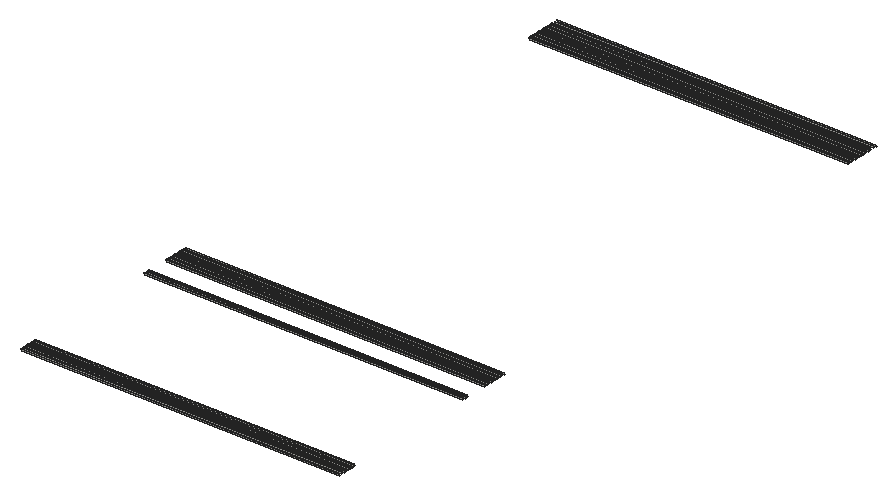
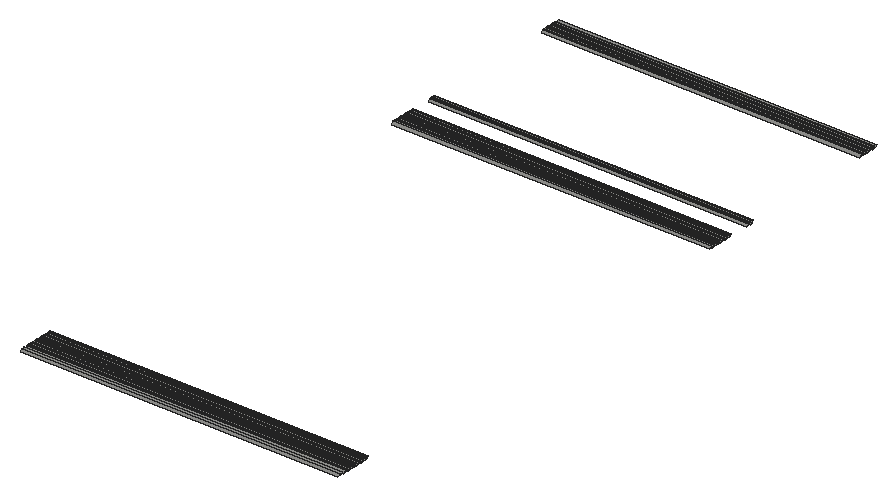
# SketchUp Ruby script. Lengths in inches.
U = 1.inch
M = Sketchup.active_model
def pt(a) = Geom::Point3d.new(a.map { |v| v * U })
def face(e, loops, mat)
  f = e.add_face(loops[0].map { |a| pt(a) })
  loops[1..].each { |l| e.add_face(l.map { |a| pt(a) }).erase! }
  f.material = f.back_material = mat if mat
  f
end
# faces: each face lists its corners as indices into pts; further lists are holes
def faces(e, pts, list, mat = nil) = list.each { |f| face(e, (f[0].is_a?(Array) ? f : [f]).map { |l| l.map { |i| pts[i] } }, mat) }
# xy, xz, yz: faces in a plane at the given z, y or x. An outline is a flat list of corners, or four numbers for a rectangle; further outlines are holes
def ring(l) = l.size == 4 ? [[l[0], l[1]], [l[2], l[1]], [l[2], l[3]], [l[0], l[3]]] : l.each_slice(2).to_a
def flat(e, list, mat, &to3) = list.each { |f| face(e, (f[0].is_a?(Array) ? f : [f]).map { |l| ring(l).map { |u, v| to3.(u, v) } }, mat) }
def xy(e, z, list, mat = nil) = flat(e, list, mat) { |x, y| [x, y, z] }
def xz(e, y, list, mat = nil) = flat(e, list, mat) { |x, z| [x, y, z] }
def yz(e, x, list, mat = nil) = flat(e, list, mat) { |y, z| [x, y, z] }
def lines(e, pts, list) = list.each { |a, b| e.add_line(pt(pts[a]), pt(pts[b])) }
# prism: a flat outline (further loops are holes) pulled along v
def prism(e, loops, v, mat = nil)
  f = face(e, loops, mat); d = Geom::Vector3d.new(v.map { |x| x * U })
  f.pushpull(f.normal.samedirection?(d) ? d.length : -d.length)
end
def box(e, o, s, mat = nil) = prism(e, [[o, [o[0] + s[0], o[1], o[2]], [o[0] + s[0], o[1] + s[1], o[2]], [o[0], o[1] + s[1], o[2]]]], [0, 0, s[2]], mat)
def at(x, y, z, deg = 0) = Geom::Transformation.translation(pt([x, y, z])) * Geom::Transformation.rotation(ORIGIN, Z_AXIS, deg.degrees)
def axes(o, x, y, z) = Geom::Transformation.new([*x, 0, *y, 0, *z, 0, *pt(o).to_a, 1])
def part(name) = M.definitions.add(name)
# library, detail: a bought-in or finely detailed component or shape, given as its bounding box
def library(name, o, s) = part(name).tap { |d| box(d.entities, o, s) }
def detail(e, o, s) = box(e.add_group.entities, o, s)
def put(e, d, t, mat = nil) = e.add_instance(d, t).tap { |i| i.material = mat if mat }
def group(e, t, mat = nil) = e.add_group.tap { |g| g.transformation = t; g.material = mat if mat }.entities
root = M.entities
c1 = part("Group452\#1")
p = [[-385.16,721.125,5.875],[385.16,721.125,5.875],[385.16,724.52,0],[-385.16,724.52,0]]
faces(c1.entities,p,[[0,1,2,3]])
c2 = part("Group453\#1")
p = [[-385.16,725.0625,5.875],[385.16,725.0625,5.875],[385.16,728.45,0],[-385.16,728.45,0]]
faces(c2.entities,p,[[0,1,2,3]])
c3 = part("Group454\#1")
p = [[-385.16,729,5.875],[385.16,729,5.875],[385.16,732.39,0],[-385.16,732.39,0]]
faces(c3.entities,p,[[0,1,2,3]])
c4 = part("Group455\#1")
p = [[-385.16,732.9375,5.875],[385.16,732.9375,5.875],[385.16,736.33,0],[-385.16,736.33,0]]
faces(c4.entities,p,[[0,1,2,3]])
c5 = part("Group456\#1")
p = [[-385.16,736.875,5.875],[385.16,736.875,5.875],[385.16,740.27,0],[-385.16,740.27,0]]
faces(c5.entities,p,[[0,1,2,3]])
c6 = part("Group457\#1")
p = [[-385.16,740.8125,5.875],[385.16,740.8125,5.875],[385.16,744.2,0],[-385.16,744.2,0]]
faces(c6.entities,p,[[0,1,2,3]])
c7 = part("Group458\#1")
p = [[385.16,748.14,0],[-385.16,748.14,0],[-385.16,744.75,5.875],[385.16,744.75,5.875]]
faces(c7.entities,p,[[0,1,2,3]])
c8 = part("Group459\#1")
p = [[-385.16,748.6875,5.875],[385.16,748.6875,5.875],[385.16,752.08,0],[-385.16,752.08,0]]
faces(c8.entities,p,[[0,1,2,3]])
c9 = part("Group460\#1")
p = [[385.16,756.02,0],[-385.16,756.02,0],[-385.16,752.625,5.875],[385.16,752.625,5.875]]
faces(c9.entities,p,[[0,1,2,3]])
c10 = part("Group461\#1")
p = [[385.16,759.95,0],[-385.16,759.95,0],[-385.16,756.5625,5.875],[385.16,756.5625,5.875]]
faces(c10.entities,p,[[0,1,2,3]])
c11 = part("Group462\#1")
p = [[-385.16,760.5,5.875],[385.16,760.5,5.875],[385.16,763.89,0],[-385.16,763.89,0]]
faces(c11.entities,p,[[0,1,2,3]])
c12 = part("Group463\#1")
p = [[-385.16,764.4375,5.875],[385.16,764.4375,5.875],[385.16,767.83,0],[-385.16,767.83,0]]
faces(c12.entities,p,[[0,1,2,3]])
c13 = part("Group464\#1")
p = [[-385.16,768.375,5.875],[385.16,768.375,5.875],[385.16,771.77,0],[-385.16,771.77,0]]
faces(c13.entities,p,[[0,1,2,3]])
c14 = part("Group465\#1")
p = [[-385.16,772.3125,5.875],[385.16,772.3125,5.875],[385.16,775.7,0],[-385.16,775.7,0]]
faces(c14.entities,p,[[0,1,2,3]])
c15 = part("Group466\#1")
p = [[385.16,779.64,0],[-385.16,779.64,0],[-385.16,776.25,5.875],[385.16,776.25,5.875]]
faces(c15.entities,p,[[0,1,2,3]])
c16 = part("Group467\#1")
p = [[385.16,783.58,0],[-385.16,783.58,0],[-385.16,780.1875,5.875],[385.16,780.1875,5.875]]
faces(c16.entities,p,[[0,1,2,3]])
c17 = part("Group468\#1")
p = [[-385.16,784.125,5.875],[385.16,784.125,5.875],[385.16,787.52,0],[-385.16,787.52,0]]
faces(c17.entities,p,[[0,1,2,3]])
c18 = part("Group469\#1")
p = [[-385.16,788.0625,5.875],[385.16,788.0625,5.875],[385.16,791.45,0],[-385.16,791.45,0]]
faces(c18.entities,p,[[0,1,2,3]])
c19 = part("Group470\#1")
p = [[-385.16,792,5.875],[385.16,792,5.875],[385.16,795.39,0],[-385.16,795.39,0]]
faces(c19.entities,p,[[0,1,2,3]])
c20 = part("Group472\#1")
p = [[385.16,803.27,0],[-385.16,803.27,0],[-385.16,799.875,5.875],[385.16,799.875,5.875]]
faces(c20.entities,p,[[0,1,2,3]])
c21 = part("Group474\#1")
p = [[-385.16,807.75,5.875],[385.16,807.75,5.875],[385.16,811.14,0],[-385.16,811.14,0]]
faces(c21.entities,p,[[0,1,2,3]])
c22 = part("Group156\#1")
p = [[385.16,-440.98,0],[-385.16,-440.98,0],[-385.16,-444.375,5.875],[385.16,-444.375,5.875]]
faces(c22.entities,p,[[0,1,2,3]])
c23 = part("Group157\#1")
p = [[-385.16,-440.4375,5.875],[385.16,-440.4375,5.875],[385.16,-437.05,0],[-385.16,-437.05,0]]
faces(c23.entities,p,[[0,1,2,3]])
c24 = part("Group158\#1")
p = [[-385.16,-436.5,5.875],[385.16,-436.5,5.875],[385.16,-433.11,0],[-385.16,-433.11,0]]
faces(c24.entities,p,[[0,1,2,3]])
c25 = part("Group159\#1")
p = [[-385.16,-432.5625,5.875],[385.16,-432.5625,5.875],[385.16,-429.17,0],[-385.16,-429.17,0]]
faces(c25.entities,p,[[0,1,2,3]])
c26 = part("Group160\#1")
p = [[385.16,-425.23,0],[-385.16,-425.23,0],[-385.16,-428.625,5.875],[385.16,-428.625,5.875]]
faces(c26.entities,p,[[0,1,2,3]])
c27 = part("Group173\#1")
p = [[-385.16,-377.4375,5.875],[385.16,-377.4375,5.875],[385.16,-374.05,0],[-385.16,-374.05,0]]
faces(c27.entities,p,[[0,1,2,3]])
c28 = part("Group174\#1")
p = [[-385.16,-373.5,5.875],[385.16,-373.5,5.875],[385.16,-370.11,0],[-385.16,-370.11,0]]
faces(c28.entities,p,[[0,1,2,3]])
c29 = part("Group175\#1")
p = [[385.16,-366.17,0],[-385.16,-366.17,0],[-385.16,-369.5625,5.875],[385.16,-369.5625,5.875]]
faces(c29.entities,p,[[0,1,2,3]])
c30 = part("Group176\#1")
p = [[-385.16,-365.625,5.875],[385.16,-365.625,5.875],[385.16,-362.23,0],[-385.16,-362.23,0]]
faces(c30.entities,p,[[0,1,2,3]])
c31 = part("Group177\#1")
p = [[385.16,-358.3,0],[-385.16,-358.3,0],[-385.16,-361.6875,5.875],[385.16,-361.6875,5.875]]
faces(c31.entities,p,[[0,1,2,3]])
c32 = part("Group178\#1")
p = [[-385.16,-357.75,5.875],[385.16,-357.75,5.875],[385.16,-354.36,0],[-385.16,-354.36,0]]
faces(c32.entities,p,[[0,1,2,3]])
c33 = part("Group179\#1")
p = [[385.16,-350.42,0],[-385.16,-350.42,0],[-385.16,-353.8125,5.875],[385.16,-353.8125,5.875]]
faces(c33.entities,p,[[0,1,2,3]])
c34 = part("Group180\#1")
p = [[385.16,-346.48,0],[-385.16,-346.48,0],[-385.16,-349.875,5.875],[385.16,-349.875,5.875]]
faces(c34.entities,p,[[0,1,2,3]])
c35 = part("Group181\#1")
p = [[-385.16,-345.9375,5.875],[385.16,-345.9375,5.875],[385.16,-342.55,0],[-385.16,-342.55,0]]
faces(c35.entities,p,[[0,1,2,3]])
c36 = part("Group182\#1")
p = [[385.16,-338.61,0],[-385.16,-338.61,0],[-385.16,-342,5.875],[385.16,-342,5.875]]
faces(c36.entities,p,[[0,1,2,3]])
c37 = part("Group183\#1")
p = [[385.16,-334.67,0],[-385.16,-334.67,0],[-385.16,-338.0625,5.875],[385.16,-338.0625,5.875]]
faces(c37.entities,p,[[0,1,2,3]])
c38 = part("Group184\#1")
p = [[-385.16,-334.125,5.875],[385.16,-334.125,5.875],[385.16,-330.73,0],[-385.16,-330.73,0]]
faces(c38.entities,p,[[0,1,2,3]])
c39 = part("Group185\#1")
p = [[-385.16,-330.1875,5.875],[385.16,-330.1875,5.875],[385.16,-326.8,0],[-385.16,-326.8,0]]
faces(c39.entities,p,[[0,1,2,3]])
c40 = part("Group186\#1")
p = [[385.16,-322.86,0],[-385.16,-322.86,0],[-385.16,-326.25,5.875],[385.16,-326.25,5.875]]
faces(c40.entities,p,[[0,1,2,3]])
c41 = part("Group187\#1")
p = [[385.16,-318.92,0],[-385.16,-318.92,0],[-385.16,-322.3125,5.875],[385.16,-322.3125,5.875]]
faces(c41.entities,p,[[0,1,2,3]])
c42 = part("Group188\#1")
p = [[-385.16,-318.375,5.875],[385.16,-318.375,5.875],[385.16,-314.98,0],[-385.16,-314.98,0]]
faces(c42.entities,p,[[0,1,2,3]])
c43 = part("Group61\#1")
p = [[-385.16,-818.4375,5.875],[385.16,-818.4375,5.875],[385.16,-815.05,0],[-385.16,-815.05,0]]
faces(c43.entities,p,[[0,1,2,3]])
c44 = part("Group63\#1")
p = [[385.16,-807.17,0],[-385.16,-807.17,0],[-385.16,-810.5625,5.875],[385.16,-810.5625,5.875]]
faces(c44.entities,p,[[0,1,2,3]])
c45 = part("Group64\#1")
p = [[385.16,-803.23,0],[-385.16,-803.23,0],[-385.16,-806.625,5.875],[385.16,-806.625,5.875]]
faces(c45.entities,p,[[0,1,2,3]])
c46 = part("Group65\#1")
p = [[385.16,-799.3,0],[-385.16,-799.3,0],[-385.16,-802.6875,5.875],[385.16,-802.6875,5.875]]
faces(c46.entities,p,[[0,1,2,3]])
c47 = part("Group66\#1")
p = [[-385.16,-798.75,5.875],[385.16,-798.75,5.875],[385.16,-795.36,0],[-385.16,-795.36,0]]
faces(c47.entities,p,[[0,1,2,3]])
c48 = part("Group67\#1")
p = [[-385.16,-794.8125,5.875],[385.16,-794.8125,5.875],[385.16,-791.42,0],[-385.16,-791.42,0]]
faces(c48.entities,p,[[0,1,2,3]])
c49 = part("Group68\#1")
p = [[385.16,-787.48,0],[-385.16,-787.48,0],[-385.16,-790.875,5.875],[385.16,-790.875,5.875]]
faces(c49.entities,p,[[0,1,2,3]])
c50 = part("Group69\#1")
p = [[385.16,-783.55,0],[-385.16,-783.55,0],[-385.16,-786.9375,5.875],[385.16,-786.9375,5.875]]
faces(c50.entities,p,[[0,1,2,3]])
c51 = part("Group70\#1")
p = [[-385.16,-783,5.875],[385.16,-783,5.875],[385.16,-779.61,0],[-385.16,-779.61,0]]
faces(c51.entities,p,[[0,1,2,3]])
c52 = part("Group71\#1")
p = [[385.16,-775.67,0],[-385.16,-775.67,0],[-385.16,-779.0625,5.875],[385.16,-779.0625,5.875]]
faces(c52.entities,p,[[0,1,2,3]])
c53 = part("Group72\#1")
p = [[385.16,-771.73,0],[-385.16,-771.73,0],[-385.16,-775.125,5.875],[385.16,-775.125,5.875]]
faces(c53.entities,p,[[0,1,2,3]])
c54 = part("Group73\#1")
p = [[385.16,-767.8,0],[-385.16,-767.8,0],[-385.16,-771.1875,5.875],[385.16,-771.1875,5.875]]
faces(c54.entities,p,[[0,1,2,3]])
put(root,c1,at(1937.93,1232.46,154.625))
put(root,c2,at(1937.93,1232.46,154.625))
put(root,c3,at(1937.93,1232.46,154.625))
put(root,c4,at(1937.93,1232.46,154.625))
put(root,c5,at(1937.93,1232.46,154.625))
put(root,c6,at(1937.93,1232.46,154.625))
put(root,c7,at(1937.93,1232.46,154.625))
put(root,c8,at(1937.93,1232.46,154.625))
put(root,c9,at(1937.93,1232.46,154.625))
put(root,c10,at(1937.93,1232.46,154.625))
put(root,c11,at(1937.93,1232.46,154.625))
put(root,c12,at(1937.93,1232.46,154.625))
put(root,c13,at(1937.93,1232.46,154.625))
put(root,c14,at(1937.93,1232.46,154.625))
put(root,c15,at(1937.93,1232.46,154.625))
put(root,c16,at(1937.93,1232.46,154.625))
put(root,c17,at(1937.93,1232.46,154.625))
put(root,c18,at(1937.93,1232.46,154.625))
put(root,c19,at(1937.93,1232.46,154.625))
put(root,c20,at(1937.93,1232.46,154.625))
put(root,c21,at(1937.93,1232.46,154.625))
put(root,c22,at(1937.93,1232.46,154.625))
put(root,c23,at(1937.93,1232.46,154.625))
put(root,c24,at(1937.93,1232.46,154.625))
put(root,c25,at(1937.93,1232.46,154.625))
put(root,c26,at(1937.93,1232.46,154.625))
put(root,c27,at(1937.93,1232.46,154.625))
put(root,c28,at(1937.93,1232.46,154.625))
put(root,c29,at(1937.93,1232.46,154.625))
put(root,c30,at(1937.93,1232.46,154.625))
put(root,c31,at(1937.93,1232.46,154.625))
put(root,c32,at(1937.93,1232.46,154.625))
put(root,c33,at(1937.93,1232.46,154.625))
put(root,c34,at(1937.93,1232.46,154.625))
put(root,c35,at(1937.93,1232.46,154.625))
put(root,c36,at(1937.93,1232.46,154.625))
put(root,c37,at(1937.93,1232.46,154.625))
put(root,c38,at(1937.93,1232.46,154.625))
put(root,c39,at(1937.93,1232.46,154.625))
put(root,c40,at(1937.93,1232.46,154.625))
put(root,c41,at(1937.93,1232.46,154.625))
put(root,c42,at(1937.93,1232.46,154.625))
put(root,c43,at(1937.93,1232.46,154.625))
put(root,c44,at(1937.93,1232.46,154.625))
put(root,c45,at(1937.93,1232.46,154.625))
put(root,c46,at(1937.93,1232.46,154.625))
put(root,c47,at(1937.93,1232.46,154.625))
put(root,c48,at(1937.93,1232.46,154.625))
put(root,c49,at(1937.93,1232.46,154.625))
put(root,c50,at(1937.93,1232.46,154.625))
put(root,c51,at(1937.93,1232.46,154.625))
put(root,c52,at(1937.93,1232.46,154.625))
put(root,c53,at(1937.93,1232.46,154.625))
put(root,c54,at(1937.93,1232.46,154.625))
